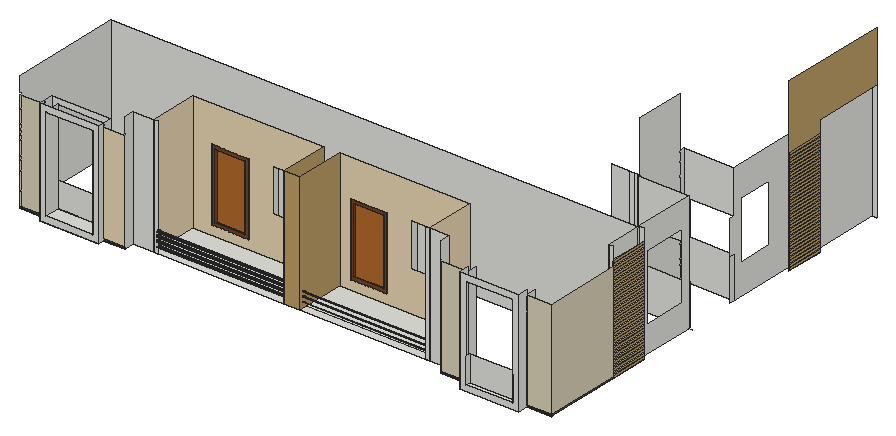
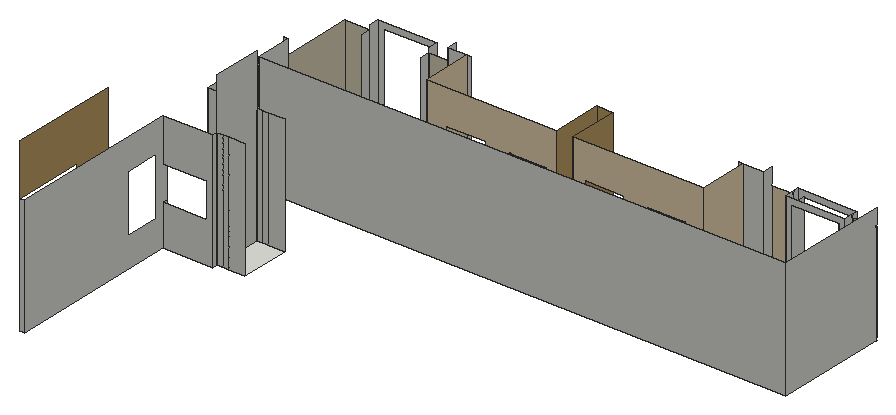
# SketchUp Ruby script. Lengths in inches.
U = 1.inch
M = Sketchup.active_model
def pt(a) = Geom::Point3d.new(a.map { |v| v * U })
def face(e, loops, mat)
  f = e.add_face(loops[0].map { |a| pt(a) })
  loops[1..].each { |l| e.add_face(l.map { |a| pt(a) }).erase! }
  f.material = f.back_material = mat if mat
  f
end
# faces: each face lists its corners as indices into pts; further lists are holes
def faces(e, pts, list, mat = nil) = list.each { |f| face(e, (f[0].is_a?(Array) ? f : [f]).map { |l| l.map { |i| pts[i] } }, mat) }
# xy, xz, yz: faces in a plane at the given z, y or x. An outline is a flat list of corners, or four numbers for a rectangle; further outlines are holes
def ring(l) = l.size == 4 ? [[l[0], l[1]], [l[2], l[1]], [l[2], l[3]], [l[0], l[3]]] : l.each_slice(2).to_a
def flat(e, list, mat, &to3) = list.each { |f| face(e, (f[0].is_a?(Array) ? f : [f]).map { |l| ring(l).map { |u, v| to3.(u, v) } }, mat) }
def xy(e, z, list, mat = nil) = flat(e, list, mat) { |x, y| [x, y, z] }
def xz(e, y, list, mat = nil) = flat(e, list, mat) { |x, z| [x, y, z] }
def yz(e, x, list, mat = nil) = flat(e, list, mat) { |y, z| [x, y, z] }
def lines(e, pts, list) = list.each { |a, b| e.add_line(pt(pts[a]), pt(pts[b])) }
# prism: a flat outline (further loops are holes) pulled along v
def prism(e, loops, v, mat = nil)
  f = face(e, loops, mat); d = Geom::Vector3d.new(v.map { |x| x * U })
  f.pushpull(f.normal.samedirection?(d) ? d.length : -d.length)
end
def box(e, o, s, mat = nil) = prism(e, [[o, [o[0] + s[0], o[1], o[2]], [o[0] + s[0], o[1] + s[1], o[2]], [o[0], o[1] + s[1], o[2]]]], [0, 0, s[2]], mat)
def at(x, y, z, deg = 0) = Geom::Transformation.translation(pt([x, y, z])) * Geom::Transformation.rotation(ORIGIN, Z_AXIS, deg.degrees)
def axes(o, x, y, z) = Geom::Transformation.new([*x, 0, *y, 0, *z, 0, *pt(o).to_a, 1])
def part(name) = M.definitions.add(name)
# library, detail: a bought-in or finely detailed component or shape, given as its bounding box
def library(name, o, s) = part(name).tap { |d| box(d.entities, o, s) }
def detail(e, o, s) = box(e.add_group.entities, o, s)
def put(e, d, t, mat = nil) = e.add_instance(d, t).tap { |i| i.material = mat if mat }
def group(e, t, mat = nil) = e.add_group.tap { |g| g.transformation = t; g.material = mat if mat }.entities
root = M.entities
M.materials.add("Generic").color = [191, 159, 103]
M.materials.add("Generic\#2").color = [235, 215, 180]
M.materials.add("Generic\#3").color = [218, 209, 183]
M.materials.add("[Color M06]").color = [86, 86, 86]
M.materials.add("[Wood Bamboo]").color = [177, 105, 43]
M.materials.add("[Wood Veneer 01]").color = [120, 70, 37]
c1 = part("Group\#5")
xy(c1.entities,0,[[0,0,1,57.75]])
xy(c1.entities,2.57,[[0,0,1,57.75]])
xz(c1.entities,0,[[0,0,1,2.57]])
xz(c1.entities,57.75,[[0,0,1,2.57]])
yz(c1.entities,1,[[0,0,57.75,2.57]])
c2 = part("Group\#6")
put(c2.entities,c1,at(0,0,4.75))
put(c2.entities,c1,at(0,0,0))
put(c2.entities,c1,at(0,0,19))
put(c2.entities,c1,at(0,0,28.5))
put(c2.entities,c1,at(0,0,133))
put(c2.entities,c1,at(0,0,152))
put(c2.entities,c1,at(0,0,128.25))
put(c2.entities,c1,at(0,0,9.5))
put(c2.entities,c1,at(0,0,123.5))
put(c2.entities,c1,at(0,0,114))
put(c2.entities,c1,at(0,0,147.25))
put(c2.entities,c1,at(0,0,118.75))
put(c2.entities,c1,at(0,0,142.5))
put(c2.entities,c1,at(0,0,109.25))
put(c2.entities,c1,at(0,0,137.75))
put(c2.entities,c1,at(0,0,104.5))
put(c2.entities,c1,at(0,0,99.75))
put(c2.entities,c1,at(0,0,95))
put(c2.entities,c1,at(0,0,85.5))
put(c2.entities,c1,at(0,0,80.75))
put(c2.entities,c1,at(0,0,90.25))
put(c2.entities,c1,at(0,0,76))
put(c2.entities,c1,at(0,0,71.25))
put(c2.entities,c1,at(0,0,38))
put(c2.entities,c1,at(0,0,14.25))
put(c2.entities,c1,at(0,0,33.25))
put(c2.entities,c1,at(0,0,57))
put(c2.entities,c1,at(0,0,23.75))
put(c2.entities,c1,at(0,0,61.75))
put(c2.entities,c1,at(0,0,156.75))
put(c2.entities,c1,at(0,0,47.5))
put(c2.entities,c1,at(0,0,52.25))
put(c2.entities,c1,at(0,0,42.75))
put(c2.entities,c1,at(0,0,66.5))
c3 = part("Group\#4")
xy(c3.entities,0,[[0,0,55.6875,6]],"[Wood Veneer 01]")
xy(c3.entities,4.75,[[4.75,0,50.9375,3]],"[Wood Veneer 01]")
xy(c3.entities,105.5,[[4.75,0,50.9375,3]],"[Wood Veneer 01]")
xy(c3.entities,110.25,[[0,0,55.6875,6]],"[Wood Veneer 01]")
xz(c3.entities,0,[[[0,0,55.6875,110.25],[4.75,4.75,50.9375,105.5]]],"[Wood Veneer 01]")
xz(c3.entities,3,[[4.75,4.75,50.9375,105.5]],"[Wood Bamboo]")
xz(c3.entities,6,[[0,0,55.6875,110.25]],"[Wood Bamboo]")
yz(c3.entities,0,[[0,0,6,110.25]],"[Wood Veneer 01]")
yz(c3.entities,4.75,[[0,4.75,3,105.5]],"[Wood Veneer 01]")
yz(c3.entities,50.9375,[[0,4.75,3,105.5]],"[Wood Veneer 01]")
yz(c3.entities,55.6875,[[0,0,6,110.25]],"[Wood Veneer 01]")
xy(root,878.32,[[682.51,53.22,771.75,68.5]])
xy(root,878.57,[[40.11,60.5625,129.35,68.5],[40.11,68.5,129.35,83.8125]])
xy(root,879,[[4.1875,68.5,40.11,69.9375],[129.35,68.5,162.33,69.9375],[641.55,68.5,682.51,69.9375],[771.75,68.5,802.875,69.9375],[802.875,68.5,809.375,69.9375],
  [807.9375,69.9375,809.375,185.01],[193.83,83.8125,391.53,158.75],[415.53,83.8125,613.23,158.75],[802.875,185.01,809.375,242.76],[684.5625,338.625,726.91,413.6875]])
xy(root,882,[[4.1875,68.5,40.11,69.9375],[129.35,68.5,162.33,69.9375],[641.55,68.5,682.51,69.9375],[682.51,68.5,771.75,83.8125],[771.75,68.5,809.375,69.9375],
  [807.9375,69.9375,809.375,185.01]])
xy(root,887.22,[[691.41,53.22,762.85,60.5625]])
xy(root,887.47,[[49.01,60.5625,120.45,83.8125]])
xy(root,892.75,[[222.01,158.75,277.69,214.75],[432.26,158.75,487.94,214.75]])
xz(root,53.22,[[[682.51,878.32,771.75,1037.71],[691.41,887.22,762.85,1028.81]]])
xz(root,60.5625,[[[40.11,878.57,129.35,1037.97],[49.01,887.47,120.45,1029.07]],[691.41,887.22,762.85,926.06]])
xz(root,68.5,[[682.51,878.32,771.75,879],[682.51,879,771.75,882]])
xz(root,68.5,[[129.35,882,162.33,1033.33]],"Generic\#2")
xz(root,68.5,[[4.1875,882,40.11,1033.33],[641.55,882,682.51,1031.12],[771.75,882,809.375,1031.12]],"Generic\#3")
xz(root,69.9375,[[4.1875,879,40.11,882],[129.35,879,162.33,882],[641.55,879,682.51,882],[771.75,879,807.9375,882]],"[Color M06]")
xz(root,83.8125,[[[40.11,878.57,129.35,1037.97],[49.01,887.47,120.45,1029.07]],[162.33,879,193.83,1059],[193.83,879,200.02,1059],[607.05,879,613.23,1059],[613.23,879,641.55,1059],
  [49.01,887.47,120.45,926.27]])
xz(root,83.8125,[[391.53,879,415.53,1059]],"Generic")
xz(root,158.75,[[[193.83,879,391.53,1059],[222.01,892.75,277.69,1003],[314.35,940.24,374.25,1006.07]],[[415.53,879,613.23,1059],[432.26,892.75,487.94,1003],[524.6,940.24,584.5,1006.07]]],"Generic\#2")
xz(root,185.01,[[802.875,879,807.9375,879,807.9375,882,809.375,882,809.375,1031.12,807.9375,1031.12,807.9375,1034.12,809.375,1034.12,809.375,1059,802.875,1059],[807.9375,879,809.375,882]])
xz(root,214.75,[[222.01,892.75,277.69,1003],[432.26,892.75,487.94,1003]])
xz(root,239.73,[[4.1875,879,802.875,1059]])
xz(root,242.76,[[802.875,879,809.375,1059]])
xz(root,335.75,[[726.91,879,802.875,879,802.875,941.3,736.34,941.3,736.34,993.42,802.875,993.42,802.875,1059,726.91,1059]])
xz(root,338.625,[[684.5625,879,709.66,1059],[709.66,879,718.29,1059],[718.29,879,726.91,1059]])
xz(root,413.6875,[[684.5625,879,709.66,1059],[709.66,879,718.29,1059],[718.29,879,726.91,1059]])
xz(root,422.3125,[[726.91,879,726.91,1059,802.875,1059,802.875,993.42,736.34,993.42,736.34,941.3,802.875,941.3,802.875,879]])
xz(root,683.8125,[[802.875,879,809.375,1059]])
yz(root,4.1875,[[69.9375,879,69.9375,882,68.5,882,68.5,1033.33,71.125,1033.33,71.125,1036.33,68.5,1036.33,68.5,1059,239.73,1059,239.73,879]])
yz(root,40.11,[[60.5625,878.57,60.5625,1037.97,68.5,1037.97,68.5,882,69.9375,882,69.9375,879,68.5,879,68.5,878.57],[68.5,878.57,83.8125,878.57,83.8125,1037.97,68.5,1037.97,68.5,1036.33,71.125,1036.33,71.125,1033.33,68.5,1033.33,68.5,882,69.9375,882,69.9375,879,68.5,879]])
yz(root,49.01,[[60.5625,887.47,83.8125,1029.07]])
yz(root,120.45,[[60.5625,887.47,83.8125,1029.07]])
yz(root,129.35,[[60.5625,878.57,68.5,878.57,68.5,879,69.9375,879,69.9375,882,68.5,882,68.5,1037.97,60.5625,1037.97],[68.5,878.57,68.5,879,69.9375,879,69.9375,882,68.5,882,68.5,1033.33,71.375,1033.33,71.375,1036.33,68.5,1036.33,68.5,1037.97,83.8125,1037.97,83.8125,878.57]])
yz(root,162.33,[[69.9375,879,69.9375,882,68.5,882,68.5,1033.33,71.375,1033.33,71.375,1036.33,68.5,1036.33,68.5,1059,83.8125,1059,83.8125,879]])
yz(root,193.83,[[[83.8125,879,158.75,1059],[90.04,910.96,89.73,911,89.44,911.12,89.2,911.31,89.01,911.55,88.89,911.84,88.85,912.15,88.89,912.45,89.01,912.74,89.2,912.99,89.44,913.17,89.73,913.29,90.04,913.33,90.35,913.29,90.63,913.17,90.88,912.99,91.07,912.74,91.18,912.45,91.23,912.15,91.18,911.84,91.07,911.55,90.88,911.31,90.63,911.12,90.35,911],[90.04,904.4,89.73,904.4375,89.44,904.56,89.2,904.74,89.01,904.99,88.89,905.28,88.85,905.58,88.89,905.89,89.01,906.18,89.2,906.42,89.44,906.61,89.73,906.73,90.04,906.77,90.35,906.73,90.63,906.61,90.88,906.42,91.07,906.18,91.18,905.89,91.23,905.58,91.18,905.28,91.07,904.99,90.88,904.74,90.63,904.56,90.35,904.4375],[90.04,897.4,89.73,897.4375,89.44,897.56,89.2,897.74,89.01,897.99,88.89,898.28,88.85,898.58,88.89,898.89,89.01,899.18,89.2,899.42,89.44,899.61,89.73,899.73,90.04,899.77,90.35,899.73,90.63,899.61,90.88,899.42,91.07,899.18,91.18,898.89,91.23,898.58,91.18,898.28,91.07,897.99,90.88,897.74,90.63,897.56,90.35,897.4375],[90.04,890.4,89.73,890.4375,89.44,890.56,89.2,890.74,89.01,890.99,88.89,891.28,88.85,891.58,88.89,891.89,89.01,892.18,89.2,892.42,89.44,892.61,89.73,892.73,90.04,892.77,90.35,892.73,90.63,892.61,90.88,892.42,91.07,892.18,91.18,891.89,91.23,891.58,91.18,891.28,91.07,890.99,90.88,890.74,90.63,890.56,90.35,890.4375],[90.04,883.71,89.73,883.75,89.44,883.87,89.2,884.06,89.01,884.3,88.89,884.59,88.85,884.9,88.89,885.2,89.01,885.49,89.2,885.74,89.44,885.92,89.73,886.04,90.04,886.08,90.35,886.04,90.63,885.92,90.88,885.74,91.07,885.49,91.18,885.2,91.23,884.9,91.18,884.59,91.07,884.3,90.88,884.06,90.63,883.87,90.35,883.75]]],"Generic\#2")
yz(root,222.01,[[158.75,892.75,214.75,1003]])
yz(root,277.69,[[158.75,892.75,214.75,1003]])
yz(root,391.53,[[[83.8125,879,158.75,1059],[90.04,910.96,90.35,911,90.63,911.12,90.88,911.31,91.07,911.55,91.18,911.84,91.23,912.15,91.18,912.45,91.07,912.74,90.88,912.99,90.63,913.17,90.35,913.29,90.04,913.33,89.73,913.29,89.44,913.17,89.2,912.99,89.01,912.74,88.89,912.45,88.85,912.15,88.89,911.84,89.01,911.55,89.2,911.31,89.44,911.12,89.73,911],[90.04,904.4,90.35,904.4375,90.63,904.56,90.88,904.74,91.07,904.99,91.18,905.28,91.23,905.58,91.18,905.89,91.07,906.18,90.88,906.42,90.63,906.61,90.35,906.73,90.04,906.77,89.73,906.73,89.44,906.61,89.2,906.42,89.01,906.18,88.89,905.89,88.85,905.58,88.89,905.28,89.01,904.99,89.2,904.74,89.44,904.56,89.73,904.4375],[90.04,897.4,90.35,897.4375,90.63,897.56,90.88,897.74,91.07,897.99,91.18,898.28,91.23,898.58,91.18,898.89,91.07,899.18,90.88,899.42,90.63,899.61,90.35,899.73,90.04,899.77,89.73,899.73,89.44,899.61,89.2,899.42,89.01,899.18,88.89,898.89,88.85,898.58,88.89,898.28,89.01,897.99,89.2,897.74,89.44,897.56,89.73,897.4375],[90.04,890.4,90.35,890.4375,90.63,890.56,90.88,890.74,91.07,890.99,91.18,891.28,91.23,891.58,91.18,891.89,91.07,892.18,90.88,892.42,90.63,892.61,90.35,892.73,90.04,892.77,89.73,892.73,89.44,892.61,89.2,892.42,89.01,892.18,88.89,891.89,88.85,891.58,88.89,891.28,89.01,890.99,89.2,890.74,89.44,890.56,89.73,890.4375],[90.04,883.71,90.35,883.75,90.63,883.87,90.88,884.06,91.07,884.3,91.18,884.59,91.23,884.9,91.18,885.2,91.07,885.49,90.88,885.74,90.63,885.92,90.35,886.04,90.04,886.08,89.73,886.04,89.44,885.92,89.2,885.74,89.01,885.49,88.89,885.2,88.85,884.9,88.89,884.59,89.01,884.3,89.2,884.06,89.44,883.87,89.73,883.75]]],"Generic")
yz(root,415.53,[[[83.8125,879,158.75,1059],[89.21,901.46,89.0625,901.48,88.93,901.54,88.8125,901.625,88.72,901.74,88.67,901.88,88.65,902.02,88.67,902.17,88.72,902.31,88.8125,902.42,88.93,902.51,89.0625,902.57,89.21,902.59,89.36,902.57,89.49,902.51,89.61,902.42,89.7,902.31,89.75,902.17,89.77,902.02,89.75,901.88,89.7,901.74,89.61,901.625,89.49,901.54,89.36,901.48],[89.21,893.96,89.0625,893.98,88.93,894.04,88.8125,894.125,88.72,894.24,88.67,894.38,88.65,894.52,88.67,894.67,88.72,894.81,88.8125,894.92,88.93,895.01,89.0625,895.07,89.21,895.09,89.36,895.07,89.49,895.01,89.61,894.92,89.7,894.81,89.75,894.67,89.77,894.52,89.75,894.38,89.7,894.24,89.61,894.125,89.49,894.04,89.36,893.98],[89.21,886.59,89.0625,886.61,88.93,886.66,88.8125,886.75,88.72,886.87,88.67,887,88.65,887.15,88.67,887.29,88.72,887.43,88.8125,887.55,88.93,887.64,89.0625,887.69,89.21,887.71,89.36,887.69,89.49,887.64,89.61,887.55,89.7,887.43,89.75,887.29,89.77,887.15,89.75,887,89.7,886.87,89.61,886.75,89.49,886.66,89.36,886.61],[89.21,916.4,89.0625,916.42,88.93,916.47,88.8125,916.5625,88.72,916.68,88.67,916.82,88.65,916.96,88.67,917.11,88.72,917.24,88.8125,917.36,88.93,917.45,89.0625,917.51,89.21,917.52,89.36,917.51,89.49,917.45,89.61,917.36,89.7,917.24,89.75,917.11,89.77,916.96,89.75,916.82,89.7,916.68,89.61,916.5625,89.49,916.47,89.36,916.42],[89.21,908.96,89.0625,908.98,88.93,909.04,88.8125,909.125,88.72,909.24,88.67,909.38,88.65,909.52,88.67,909.67,88.72,909.81,88.8125,909.92,88.93,910.01,89.0625,910.07,89.21,910.09,89.36,910.07,89.49,910.01,89.61,909.92,89.7,909.81,89.75,909.67,89.77,909.52,89.75,909.38,89.7,909.24,89.61,909.125,89.49,909.04,89.36,908.98]]],"Generic")
yz(root,432.26,[[158.75,892.75,214.75,1003]])
yz(root,487.94,[[158.75,892.75,214.75,1003]])
yz(root,607.05,[[89.21,886.59,89.36,886.61,89.49,886.66,89.61,886.75,89.7,886.87,89.75,887,89.77,887.15,89.75,887.29,89.7,887.43,89.61,887.55,89.49,887.64,89.36,887.69,89.21,887.71,89.0625,887.69,88.93,887.64,88.8125,887.55,88.72,887.43,88.67,887.29,88.65,887.15,88.67,887,88.72,886.87,88.8125,886.75,88.93,886.66,89.0625,886.61],[89.21,893.96,89.36,893.98,89.49,894.04,89.61,894.125,89.7,894.24,89.75,894.38,89.77,894.52,89.75,894.67,89.7,894.81,89.61,894.92,89.49,895.01,89.36,895.07,89.21,895.09,89.0625,895.07,88.93,895.01,88.8125,894.92,88.72,894.81,88.67,894.67,88.65,894.52,88.67,894.38,88.72,894.24,88.8125,894.125,88.93,894.04,89.0625,893.98],[89.21,901.46,89.36,901.48,89.49,901.54,89.61,901.625,89.7,901.74,89.75,901.88,89.77,902.02,89.75,902.17,89.7,902.31,89.61,902.42,89.49,902.51,89.36,902.57,89.21,902.59,89.0625,902.57,88.93,902.51,88.8125,902.42,88.72,902.31,88.67,902.17,88.65,902.02,88.67,901.88,88.72,901.74,88.8125,901.625,88.93,901.54,89.0625,901.48]])
yz(root,613.23,[[83.8125,879,158.75,1059]],"Generic\#2")
yz(root,641.55,[[69.9375,879,83.8125,879,83.8125,1059,68.5,1059,68.5,1034.12,69.9375,1034.12,69.9375,1031.12,68.5,1031.12,68.5,882,69.9375,882]])
yz(root,682.51,[[53.22,878.32,68.5,1037.71],[68.5,879,69.9375,882],[68.5,882,83.8125,1031.12]])
yz(root,691.41,[[53.22,887.22,60.5625,926.06]])
yz(root,726.91,[[335.75,879,338.625,1059],[338.625,879,413.6875,1136.625],[413.6875,879,422.3125,1059]])
yz(root,762.85,[[53.22,887.22,60.5625,926.06]])
yz(root,771.75,[[53.22,878.32,68.5,1037.71],[68.5,879,69.9375,882],[68.5,882,83.8125,1031.12]])
yz(root,802.875,[[185.01,879,239.73,1059],[239.73,879,242.76,1059],[[242.76,879,335.75,1059],[257.24,918.09,324.36,1018.78]],[335.75,879,338.625,941.3],[413.6875,879,422.3125,941.3],
  [[422.3125,879,422.3125,941.3,413.6875,941.3,413.6875,993.42,422.3125,993.42,422.3125,1059,683.8125,1059,683.8125,879],[434.88,924.5,489.19,1012.38]]])
yz(root,807.9375,[[69.9375,879,185.01,882]],"[Color M06]")
yz(root,809.375,[[185.01,879,242.76,1037.39]])
yz(root,809.375,[[518.09,879,575.84,879,575.84,1059,683.8125,1059,683.8125,1136.625,518.09,1136.625]],"Generic")
yz(root,809.375,[[68.5,882,185.01,1031.12]],"Generic\#3")
p = [[193.83,89.44,883.87],[193.83,89.73,883.75],[391.53,89.73,883.75],[391.53,89.44,883.87],[193.83,90.04,883.71],[391.53,90.04,883.71],
  [193.83,90.35,883.75],[391.53,90.35,883.75],[193.83,90.63,883.87],[391.53,90.63,883.87],[193.83,89.2,884.06],[391.53,89.2,884.06],
  [193.83,90.88,884.06],[391.53,90.88,884.06],[193.83,89.01,884.3],[391.53,89.01,884.3],[193.83,91.07,884.3],[391.53,91.07,884.3],
  [193.83,88.89,884.59],[391.53,88.89,884.59],[193.83,91.18,884.59],[391.53,91.18,884.59],[193.83,88.85,884.9],[391.53,88.85,884.9],
  [193.83,91.23,884.9],[391.53,91.23,884.9],[193.83,88.89,885.2],[391.53,88.89,885.2],[193.83,91.18,885.2],[391.53,91.18,885.2],
  [193.83,89.01,885.49],[391.53,89.01,885.49],[193.83,91.07,885.49],[391.53,91.07,885.49],[193.83,89.2,885.74],[391.53,89.2,885.74],
  [193.83,90.88,885.74],[391.53,90.88,885.74],[193.83,89.44,885.92],[391.53,89.44,885.92],[193.83,90.63,885.92],[391.53,90.63,885.92],
  [193.83,89.73,886.04],[391.53,89.73,886.04],[193.83,90.35,886.04],[391.53,90.35,886.04],[193.83,90.04,886.08],[391.53,90.04,886.08],
  [415.53,88.93,886.66],[415.53,89.0625,886.61],[607.05,89.0625,886.61],[607.05,88.93,886.66],[415.53,89.21,886.59],[607.05,89.21,886.59],
  [415.53,89.36,886.61],[607.05,89.36,886.61],[415.53,89.49,886.66],[607.05,89.49,886.66],[415.53,88.8125,886.75],[607.05,88.8125,886.75],
  [415.53,89.61,886.75],[607.05,89.61,886.75],[415.53,88.72,886.87],[607.05,88.72,886.87],[415.53,89.7,886.87],[607.05,89.7,886.87],
  [415.53,88.67,887],[607.05,88.67,887],[415.53,89.75,887],[607.05,89.75,887],[415.53,88.65,887.15],[607.05,88.65,887.15],
  [415.53,89.77,887.15],[607.05,89.77,887.15],[415.53,88.67,887.29],[607.05,88.67,887.29],[415.53,89.75,887.29],[607.05,89.75,887.29],
  [415.53,88.72,887.43],[607.05,88.72,887.43],[415.53,89.7,887.43],[607.05,89.7,887.43],[415.53,88.8125,887.55],[607.05,88.8125,887.55],
  [415.53,89.61,887.55],[607.05,89.61,887.55],[415.53,88.93,887.64],[607.05,88.93,887.64],[415.53,89.49,887.64],[607.05,89.49,887.64],
  [415.53,89.0625,887.69],[607.05,89.0625,887.69],[415.53,89.36,887.69],[607.05,89.36,887.69],[415.53,89.21,887.71],[607.05,89.21,887.71],
  [193.83,89.44,890.56],[193.83,89.73,890.4375],[391.53,89.73,890.4375],[391.53,89.44,890.56],[193.83,90.04,890.4],[391.53,90.04,890.4],
  [193.83,90.35,890.4375],[391.53,90.35,890.4375],[193.83,90.63,890.56],[391.53,90.63,890.56],[193.83,89.2,890.74],[391.53,89.2,890.74],
  [193.83,90.88,890.74],[391.53,90.88,890.74],[193.83,89.01,890.99],[391.53,89.01,890.99],[193.83,91.07,890.99],[391.53,91.07,890.99],
  [193.83,88.89,891.28],[391.53,88.89,891.28],[193.83,91.18,891.28],[391.53,91.18,891.28],[193.83,88.85,891.58],[391.53,88.85,891.58],
  [193.83,91.23,891.58],[391.53,91.23,891.58],[193.83,88.89,891.89],[391.53,88.89,891.89],[193.83,91.18,891.89],[391.53,91.18,891.89],
  [193.83,89.01,892.18],[391.53,89.01,892.18],[193.83,91.07,892.18],[391.53,91.07,892.18],[193.83,89.2,892.42],[391.53,89.2,892.42],
  [193.83,90.88,892.42],[391.53,90.88,892.42],[193.83,89.44,892.61],[391.53,89.44,892.61],[193.83,90.63,892.61],[391.53,90.63,892.61],
  [193.83,89.73,892.73],[391.53,89.73,892.73],[193.83,90.35,892.73],[391.53,90.35,892.73],[193.83,90.04,892.77],[391.53,90.04,892.77],
  [415.53,88.8125,894.125],[415.53,88.93,894.04],[607.05,88.93,894.04],[607.05,88.8125,894.125],[415.53,89.0625,893.98],[607.05,89.0625,893.98],
  [415.53,89.21,893.96],[607.05,89.21,893.96],[415.53,89.36,893.98],[607.05,89.36,893.98],[415.53,89.49,894.04],[607.05,89.49,894.04],
  [415.53,89.61,894.125],[607.05,89.61,894.125],[415.53,88.72,894.24],[607.05,88.72,894.24],[415.53,89.7,894.24],[607.05,89.7,894.24],
  [415.53,88.67,894.38],[607.05,88.67,894.38],[415.53,89.75,894.38],[607.05,89.75,894.38],[415.53,88.65,894.52],[607.05,88.65,894.52],
  [415.53,89.77,894.52],[607.05,89.77,894.52],[415.53,88.67,894.67],[607.05,88.67,894.67],[415.53,89.75,894.67],[607.05,89.75,894.67],
  [415.53,88.72,894.81],[607.05,88.72,894.81],[415.53,89.7,894.81],[607.05,89.7,894.81],[415.53,88.8125,894.92],[607.05,88.8125,894.92],
  [415.53,89.61,894.92],[607.05,89.61,894.92],[415.53,88.93,895.01],[607.05,88.93,895.01],[415.53,89.49,895.01],[607.05,89.49,895.01],
  [415.53,89.0625,895.07],[607.05,89.0625,895.07],[415.53,89.36,895.07],[607.05,89.36,895.07],[415.53,89.21,895.09],[607.05,89.21,895.09],
  [193.83,89.44,897.56],[193.83,89.73,897.4375],[391.53,89.73,897.4375],[391.53,89.44,897.56],[193.83,90.04,897.4],[391.53,90.04,897.4],
  [193.83,90.35,897.4375],[391.53,90.35,897.4375],[193.83,90.63,897.56],[391.53,90.63,897.56],[193.83,89.2,897.74],[391.53,89.2,897.74],
  [193.83,90.88,897.74],[391.53,90.88,897.74],[193.83,89.01,897.99],[391.53,89.01,897.99],[193.83,91.07,897.99],[391.53,91.07,897.99],
  [193.83,88.89,898.28],[391.53,88.89,898.28],[193.83,91.18,898.28],[391.53,91.18,898.28],[193.83,88.85,898.58],[391.53,88.85,898.58],
  [193.83,91.23,898.58],[391.53,91.23,898.58],[193.83,88.89,898.89],[391.53,88.89,898.89],[193.83,91.18,898.89],[391.53,91.18,898.89],
  [193.83,89.01,899.18],[391.53,89.01,899.18],[193.83,91.07,899.18],[391.53,91.07,899.18],[193.83,89.2,899.42],[391.53,89.2,899.42],
  [193.83,90.88,899.42],[391.53,90.88,899.42],[193.83,89.44,899.61],[391.53,89.44,899.61],[193.83,90.63,899.61],[391.53,90.63,899.61],
  [193.83,89.73,899.73],[391.53,89.73,899.73],[193.83,90.35,899.73],[391.53,90.35,899.73],[193.83,90.04,899.77],[391.53,90.04,899.77],
  [415.53,88.8125,901.625],[415.53,88.93,901.54],[607.05,88.93,901.54],[607.05,88.8125,901.625],[415.53,89.0625,901.48],[607.05,89.0625,901.48],
  [415.53,89.21,901.46],[607.05,89.21,901.46],[415.53,89.36,901.48],[607.05,89.36,901.48],[415.53,89.49,901.54],[607.05,89.49,901.54],
  [415.53,89.61,901.625],[607.05,89.61,901.625],[415.53,88.72,901.74],[607.05,88.72,901.74],[415.53,89.7,901.74],[607.05,89.7,901.74],
  [415.53,88.67,901.88],[607.05,88.67,901.88],[415.53,89.75,901.88],[607.05,89.75,901.88],[415.53,88.65,902.02],[607.05,88.65,902.02],
  [415.53,89.77,902.02],[607.05,89.77,902.02],[415.53,88.67,902.17],[607.05,88.67,902.17],[415.53,89.75,902.17],[607.05,89.75,902.17],
  [415.53,88.72,902.31],[607.05,88.72,902.31],[415.53,89.7,902.31],[607.05,89.7,902.31],[415.53,88.8125,902.42],[607.05,88.8125,902.42],
  [415.53,89.61,902.42],[607.05,89.61,902.42],[415.53,88.93,902.51],[607.05,88.93,902.51],[415.53,89.49,902.51],[607.05,89.49,902.51],
  [415.53,89.0625,902.57],[607.05,89.0625,902.57],[415.53,89.36,902.57],[607.05,89.36,902.57],[415.53,89.21,902.59],[607.05,89.21,902.59],
  [193.83,89.44,904.56],[193.83,89.73,904.4375],[391.53,89.73,904.4375],[391.53,89.44,904.56],[193.83,90.04,904.4],[391.53,90.04,904.4],
  [193.83,90.35,904.4375],[391.53,90.35,904.4375],[193.83,90.63,904.56],[391.53,90.63,904.56],[193.83,89.2,904.74],[391.53,89.2,904.74],
  [193.83,90.88,904.74],[391.53,90.88,904.74],[193.83,89.01,904.99],[391.53,89.01,904.99],[193.83,91.07,904.99],[391.53,91.07,904.99],
  [193.83,88.89,905.28],[391.53,88.89,905.28],[193.83,91.18,905.28],[391.53,91.18,905.28],[193.83,88.85,905.58],[391.53,88.85,905.58],
  [193.83,91.23,905.58],[391.53,91.23,905.58],[193.83,88.89,905.89],[391.53,88.89,905.89],[193.83,91.18,905.89],[391.53,91.18,905.89],
  [193.83,89.01,906.18],[391.53,89.01,906.18],[193.83,91.07,906.18],[391.53,91.07,906.18],[193.83,89.2,906.42],[391.53,89.2,906.42],
  [193.83,90.88,906.42],[391.53,90.88,906.42],[193.83,89.44,906.61],[391.53,89.44,906.61],[193.83,90.63,906.61],[391.53,90.63,906.61],
  [193.83,89.73,906.73],[391.53,89.73,906.73],[193.83,90.35,906.73],[391.53,90.35,906.73],[193.83,90.04,906.77],[391.53,90.04,906.77],
  [415.53,95.8125,879],[607.05,95.8125,879],[415.53,89.21,887.18],[613.23,89.21,887.18],[415.53,89.21,902.06],[613.23,89.21,902.06],
  [415.53,89.21,894.62],[613.23,89.21,894.62],[193.83,90.04,905.4],[391.53,90.04,905.4],[193.83,90.04,885.15],[391.53,90.04,885.15],
  [193.83,90.04,898.65],[391.53,90.04,898.65],[193.83,90.04,891.9],[391.53,90.04,891.9],[809.375,335.75,879],[802.875,335.75,879],
  [802.875,69.9375,879],[802.875,185.01,879]]
faces(root,p,[[0,1,2,3],[1,4,5,2],[4,6,7,5],[6,8,9,7],[10,0,3,11],[8,12,13,9],[14,10,11,15],[12,16,17,13],
  [18,14,15,19],[16,20,21,17],[22,18,19,23],[20,24,25,21],[26,22,23,27],[24,28,29,25],[30,26,27,31],[28,32,33,29],
  [34,30,31,35],[32,36,37,33],[38,34,35,39],[36,40,41,37],[42,38,39,43],[40,44,45,41],[46,42,43,47],[44,46,47,45],
  [48,49,50,51],[49,52,53,50],[52,54,55,53],[54,56,57,55],[58,48,51,59],[56,60,61,57],[62,58,59,63],[60,64,65,61],
  [66,62,63,67],[64,68,69,65],[70,66,67,71],[68,72,73,69],[74,70,71,75],[72,76,77,73],[78,74,75,79],[76,80,81,77],
  [82,78,79,83],[80,84,85,81],[86,82,83,87],[84,88,89,85],[90,86,87,91],[88,92,93,89],[94,90,91,95],[92,94,95,93],
  [96,97,98,99],[97,100,101,98],[100,102,103,101],[102,104,105,103],[106,96,99,107],[104,108,109,105],[110,106,107,111],[108,112,113,109],
  [114,110,111,115],[112,116,117,113],[118,114,115,119],[116,120,121,117],[122,118,119,123],[120,124,125,121],[126,122,123,127],[124,128,129,125],
  [130,126,127,131],[128,132,133,129],[134,130,131,135],[132,136,137,133],[138,134,135,139],[136,140,141,137],[142,138,139,143],[140,142,143,141],
  [144,145,146,147],[145,148,149,146],[148,150,151,149],[150,152,153,151],[152,154,155,153],[154,156,157,155],[158,144,147,159],[156,160,161,157],
  [162,158,159,163],[160,164,165,161],[166,162,163,167],[164,168,169,165],[170,166,167,171],[168,172,173,169],[174,170,171,175],[172,176,177,173],
  [178,174,175,179],[176,180,181,177],[182,178,179,183],[180,184,185,181],[186,182,183,187],[184,188,189,185],[190,186,187,191],[188,190,191,189],
  [192,193,194,195],[193,196,197,194],[196,198,199,197],[198,200,201,199],[202,192,195,203],[200,204,205,201],[206,202,203,207],[204,208,209,205],
  [210,206,207,211],[208,212,213,209],[214,210,211,215],[212,216,217,213],[218,214,215,219],[216,220,221,217],[222,218,219,223],[220,224,225,221],
  [226,222,223,227],[224,228,229,225],[230,226,227,231],[228,232,233,229],[234,230,231,235],[232,236,237,233],[238,234,235,239],[236,238,239,237],
  [240,241,242,243],[241,244,245,242],[244,246,247,245],[246,248,249,247],[248,250,251,249],[250,252,253,251],[254,240,243,255],[252,256,257,253],
  [258,254,255,259],[256,260,261,257],[262,258,259,263],[260,264,265,261],[266,262,263,267],[264,268,269,265],[270,266,267,271],[268,272,273,269],
  [274,270,271,275],[272,276,277,273],[278,274,275,279],[276,280,281,277],[282,278,279,283],[280,284,285,281],[286,282,283,287],[284,286,287,285],
  [288,289,290,291],[289,292,293,290],[292,294,295,293],[294,296,297,295],[298,288,291,299],[296,300,301,297],[302,298,299,303],[300,304,305,301],
  [306,302,303,307],[304,308,309,305],[310,306,307,311],[308,312,313,309],[314,310,311,315],[312,316,317,313],[318,314,315,319],[316,320,321,317],
  [322,318,319,323],[320,324,325,321],[326,322,323,327],[324,328,329,325],[330,326,327,331],[328,332,333,329],[334,330,331,335],[332,334,335,333]])
lines(root,p,[[336,337],[338,339],[340,341],[342,343],[344,345],[346,347],[348,349],[350,351],[352,353],[354,355]])
put(root,c2,at(809.375,185.01,880.64),"Generic")
put(root,c2,at(809.375,518.09,880.64),"Generic")
put(root,c3,at(432.26,158.75,892.75))
put(root,c3,at(222.01,158.75,892.75))
